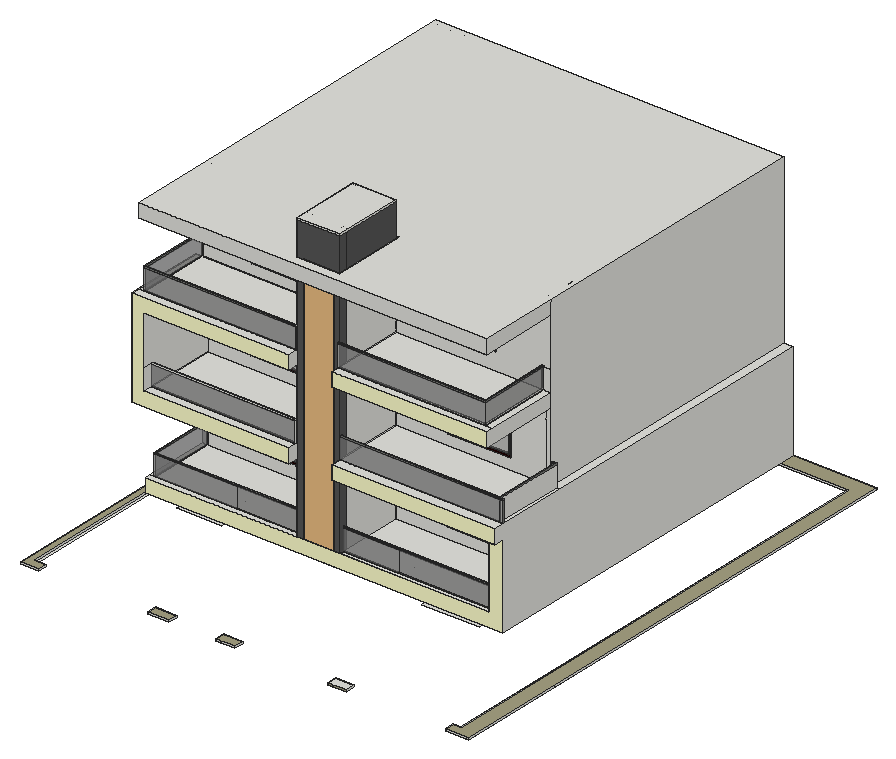
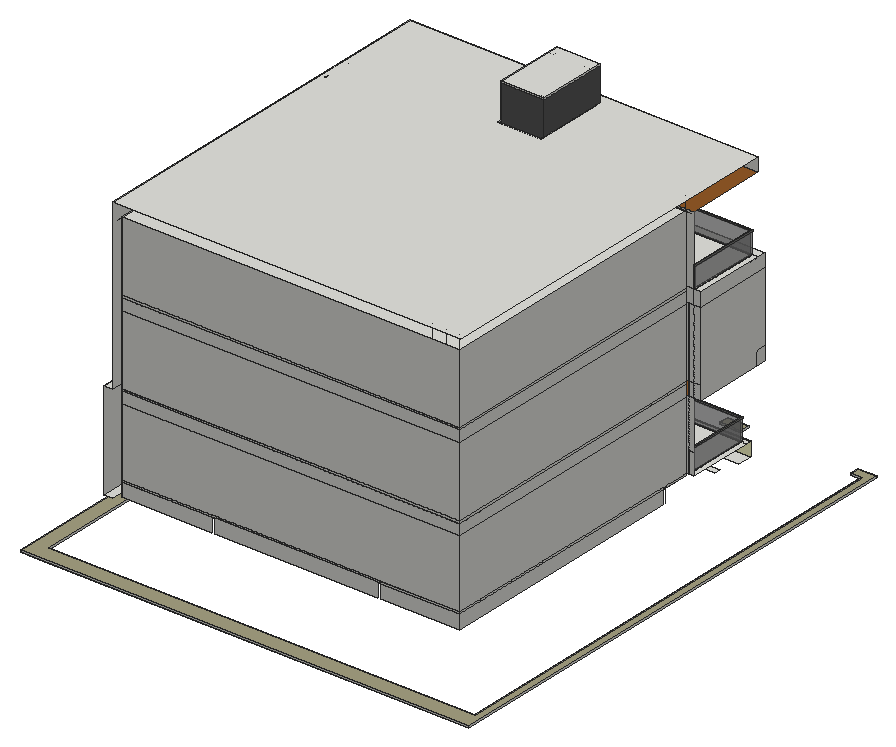
# SketchUp Ruby script. Lengths in inches.
U = 1.inch
M = Sketchup.active_model
def pt(a) = Geom::Point3d.new(a.map { |v| v * U })
def face(e, loops, mat)
  f = e.add_face(loops[0].map { |a| pt(a) })
  loops[1..].each { |l| e.add_face(l.map { |a| pt(a) }).erase! }
  f.material = f.back_material = mat if mat
  f
end
# faces: each face lists its corners as indices into pts; further lists are holes
def faces(e, pts, list, mat = nil) = list.each { |f| face(e, (f[0].is_a?(Array) ? f : [f]).map { |l| l.map { |i| pts[i] } }, mat) }
# xy, xz, yz: faces in a plane at the given z, y or x. An outline is a flat list of corners, or four numbers for a rectangle; further outlines are holes
def ring(l) = l.size == 4 ? [[l[0], l[1]], [l[2], l[1]], [l[2], l[3]], [l[0], l[3]]] : l.each_slice(2).to_a
def flat(e, list, mat, &to3) = list.each { |f| face(e, (f[0].is_a?(Array) ? f : [f]).map { |l| ring(l).map { |u, v| to3.(u, v) } }, mat) }
def xy(e, z, list, mat = nil) = flat(e, list, mat) { |x, y| [x, y, z] }
def xz(e, y, list, mat = nil) = flat(e, list, mat) { |x, z| [x, y, z] }
def yz(e, x, list, mat = nil) = flat(e, list, mat) { |y, z| [x, y, z] }
def lines(e, pts, list) = list.each { |a, b| e.add_line(pt(pts[a]), pt(pts[b])) }
# prism: a flat outline (further loops are holes) pulled along v
def prism(e, loops, v, mat = nil)
  f = face(e, loops, mat); d = Geom::Vector3d.new(v.map { |x| x * U })
  f.pushpull(f.normal.samedirection?(d) ? d.length : -d.length)
end
def box(e, o, s, mat = nil) = prism(e, [[o, [o[0] + s[0], o[1], o[2]], [o[0] + s[0], o[1] + s[1], o[2]], [o[0], o[1] + s[1], o[2]]]], [0, 0, s[2]], mat)
def at(x, y, z, deg = 0) = Geom::Transformation.translation(pt([x, y, z])) * Geom::Transformation.rotation(ORIGIN, Z_AXIS, deg.degrees)
def axes(o, x, y, z) = Geom::Transformation.new([*x, 0, *y, 0, *z, 0, *pt(o).to_a, 1])
def part(name) = M.definitions.add(name)
# library, detail: a bought-in or finely detailed component or shape, given as its bounding box
def library(name, o, s) = part(name).tap { |d| box(d.entities, o, s) }
def detail(e, o, s) = box(e.add_group.entities, o, s)
def put(e, d, t, mat = nil) = e.add_instance(d, t).tap { |i| i.material = mat if mat }
def group(e, t, mat = nil) = e.add_group.tap { |g| g.transformation = t; g.material = mat if mat }.entities
root = M.entities
M.materials.add("[Color A08]").color = [30, 0, 0]
M.materials.add("[Color E01]").color = [255, 255, 204]
M.materials.add("[Color M06]").color = [86, 86, 86]
M.materials.add("[Metal Seamed]").color = [118, 119, 115]
M.materials.add("[Stone Coursed Rough]").color = [165, 160, 130]
M.materials.add("[Translucent Glass Gray]").color = [128, 128, 128]
M.materials["[Translucent Glass Gray]"].alpha = 0.5
M.materials.add("[Wood Floor Parquet]").color = [145, 89, 39]
c1 = library("Group\#4",[0,0,0],[132.0625,6,363.3125])
c2 = part("Group\#3")
xy(c2.entities,0,[[0,0,60.375,4]])
xy(c2.entities,4.67,[[4.67,0,28.45,4],[32.75,0,55.71,4]],"[Color A08]")
xy(c2.entities,93.02,[[4.67,0,28.45,4],[32.75,0,55.71,4]])
xy(c2.entities,97.6875,[[0,0,60.375,4]],"[Color A08]")
xz(c2.entities,0,[[[0,0,60.375,97.6875],[4.67,4.67,28.45,93.02],[32.75,4.67,55.71,93.02]]],"[Color A08]")
xz(c2.entities,0,[[4.67,4.67,28.45,93.02],[32.75,4.67,55.71,93.02]],"[Translucent Glass Gray]")
xz(c2.entities,4,[[[0,0,60.375,97.6875],[4.67,4.67,28.45,93.02],[32.75,4.67,55.71,93.02]]],"[Color A08]")
yz(c2.entities,0,[[0,0,4,97.6875]],"[Color A08]")
yz(c2.entities,4.67,[[0,4.67,4,93.02]],"[Color A08]")
yz(c2.entities,28.45,[[0,4.67,4,93.02]],"[Color A08]")
yz(c2.entities,32.75,[[0,4.67,4,93.02]],"[Color A08]")
yz(c2.entities,55.71,[[0,4.67,4,93.02]],"[Color A08]")
yz(c2.entities,60.375,[[0,0,4,97.6875]],"[Color A08]")
c3 = part("Group\#2")
xy(c3.entities,0,[[0,0,95.3125,6]])
xy(c3.entities,4.01,[[4.01,0,28.72,6],[32.91,0,56.47,6],[60.66,0,91.31,6]],"[Color A08]")
xy(c3.entities,82.62,[[4.01,0,28.72,6],[32.91,0,56.47,6],[60.66,0,91.31,6]])
xy(c3.entities,86.625,[[0,0,95.3125,6]],"[Color A08]")
xz(c3.entities,0,[[[0,0,95.3125,86.625],[60.66,4.01,91.31,82.62],[4.01,4.01,28.72,82.62],[32.91,4.01,56.47,82.62]]],"[Color A08]")
xz(c3.entities,0,[[4.01,4.01,28.72,82.62],[32.91,4.01,56.47,82.62],[60.66,4.01,91.31,82.62]],"[Translucent Glass Gray]")
xz(c3.entities,6,[[[0,0,95.3125,86.625],[60.66,4.01,91.31,82.62],[4.01,4.01,28.72,82.62],[32.91,4.01,56.47,82.62]]],"[Color A08]")
yz(c3.entities,0,[[0,0,6,86.625]],"[Color A08]")
yz(c3.entities,4.01,[[0,4.01,6,82.62]],"[Color A08]")
yz(c3.entities,28.72,[[0,4.01,6,82.62]],"[Color A08]")
yz(c3.entities,32.91,[[0,4.01,6,82.62]],"[Color A08]")
yz(c3.entities,56.47,[[0,4.01,6,82.62]],"[Color A08]")
yz(c3.entities,60.66,[[0,4.01,6,82.62]],"[Color A08]")
yz(c3.entities,91.31,[[0,4.01,6,82.62]],"[Color A08]")
yz(c3.entities,95.3125,[[0,0,6,86.625]],"[Color A08]")
xy(root,126,[[0,0,0,878.5,746.625,878.5,746.625,849.54,11.8,849.54,11.8,16.17,31.52,16.17,31.52,0],[219.71,0,256.64,16.17],[336.85,0,370.02,16.17],[529.83,0,562.05,16.17],[732.77,0,732.77,16.17,746.625,16.17,746.625,183.0625,772,183.0625,772,0],
  [11.8,16.17,16.36,849.54],[746.625,183.0625,772,849.54],[746.625,849.54,772,878.5]])
xy(root,129,[[529.83,0,562.05,16.17]])
xy(root,129,[[0,0,31.52,0,31.52,16.17,11.8,16.17,11.8,849.54,746.625,849.54,746.625,16.17,732.77,16.17,732.77,0,772,0,772,878.5,0,878.5],[219.71,0,256.64,16.17],[336.85,0,370.02,16.17]],"[Stone Coursed Rough]")
xy(root,160.875,[[269.59,330.0625,317.59,336.0625],[446.24,330.0625,494.24,336.0625]])
xy(root,174.47,[[362.91,203.5,408.97,209.5625]])
xy(root,174.78,[[545.68,183.0625,644.56,192.0625]])
xy(root,175.07,[[124.03,183.0625,201.03,192.0625]])
xy(root,196.875,[[89.625,159.1875,239.625,183.0625],[348.1875,159.1875,360.82,183.0625],[360.82,159.1875,360.82,192.0625,348.1875,192.0625,348.1875,203.5,422.35,203.5,422.35,192.0625,412.84,192.0625,412.84,159.1875],[412.84,159.1875,422.35,183.0625],[519.875,159.1875,704.125,183.0625],
  [689.625,183.0625,704.125,783.0625]])
xy(root,196.875,[[239.625,159.1875,348.1875,330.0625],[422.35,159.1875,519.875,330.0625]],"[Wood Floor Parquet]")
xy(root,220.875,[[89.625,159.1875,348.1875,166.875],[348.1875,159.1875,360.82,175.5625],[360.82,159.1875,412.84,168.1875],[412.84,159.1875,422.35,159.1875,412.84,161.125],[422.35,159.1875,680.625,159.1875,680.625,165.3,422.36,165.72],
  [680.625,165.3,422.36,165.72,422.37,168.1875,680.625,168.1875],[89.625,166.875,97,281.125],[97,166.875,97,281.125,98.625,281.125,98.625,168.1875,348.1875,168.1875,348.1875,166.875],[98.625,168.1875,348.1875,281.125],[360.82,168.1875,412.84,178.89],
  [422.37,168.1875,680.625,168.1875,680.625,281.125,422.38,281.125,422.38,175.5625],[348.1875,175.5625,348.1875,281.125,418.5,281.125,418.5,277.79,351.52,277.79,351.52,178.89,360.82,178.89,360.82,175.5625],[412.84,175.5625,412.84,178.89,419.05,178.89,419.05,277.79,418.5,277.79,418.5,281.125,422.38,281.125,422.38,175.5625],[351.52,178.89,419.05,277.79],[348.1875,281.125,351.23,287.125],
  [351.23,281.125,418.5,287.125],[418.5,281.125,422.38,287.125],[98.625,287.125,98.625,774.0625,680.625,774.0625,680.625,287.125,418.5,287.125,418.5,336.0625,351.23,336.0625,351.23,287.125],[351.23,287.125,418.5,336.0625]])
xy(root,223.875,[[98.625,287.125,680.625,774.0625]])
xy(root,233.21,[[370.73,277.79,406.73,284.92]])
xy(root,238.59,[[511.46,281.125,620.96,287.125]])
xy(root,242.34,[[172.09,281.125,281.59,287.125]])
xy(root,256.875,[[680.625,165.3,422.36,165.72,422.37,168.1875,680.625,168.1875],[97,166.875,97,281.125,98.625,281.125,98.625,168.1875,348.1875,168.1875,348.1875,166.875]])
xy(root,258.875,[[680.625,165.3,680.625,168.1875,422.37,168.1875,422.36,165.72],[97,166.875,348.1875,166.875,348.1875,168.1875,98.625,168.1875,98.625,281.125,97,281.125]],"[Metal Seamed]")
xy(root,317.21,[[370.73,277.79,406.73,284.92]])
xy(root,320.22,[[511.46,281.125,620.96,287.125]])
xy(root,323.97,[[172.09,281.125,281.59,287.125]])
xy(root,340.875,[[78.1875,142.25,78.1875,159.1875,98.625,159.1875,98.625,281.125,348.1875,281.125,348.1875,142.25],[422.38,142.25,422.38,281.125,680.625,281.125,680.625,159.1875,704.125,159.1875,704.125,142.25],[78.1875,159.1875,89.625,281.125],[89.625,159.1875,98.625,281.125]],"[Wood Floor Parquet]")
xy(root,360.875,[[98.625,287.125,680.625,774.0625]])
xy(root,364.875,[[98.625,142.25,348.1875,156.75],[422.38,142.25,704.125,159.3125],[98.625,156.75,348.1875,159.1875],[98.625,159.1875,348.1875,281.125],[422.38,159.3125,704.125,161],
  [422.38,161,696.47,281.125],[696.47,161,696.47,281.125,689.625,281.125,689.625,282.2,698.1875,282.2,698.1875,161],[698.1875,161,704.125,283.32],[689.625,282.2,698.1875,282.2,698.1875,283.32,704.125,283.32,704.125,783.0625,689.625,783.0625],[98.625,287.125,680.625,774.0625]])
xy(root,383.59,[[172.09,281.125,281.59,287.125],[511.46,281.125,620.96,287.125]])
xy(root,390.46,[[370.73,277.79,406.73,286.23]])
xy(root,400.875,[[98.625,156.75,348.1875,159.1875],[422.38,159.3125,704.125,161],[696.47,161,696.47,281.125,689.625,281.125,689.625,282.2,698.1875,282.2,698.1875,161]])
xy(root,402.875,[[98.625,156.75,348.1875,159.1875]])
xy(root,402.875,[[422.38,159.3125,704.125,161],[696.47,161,698.1875,161,698.1875,282.2,689.625,282.2,689.625,281.125,696.47,281.125]],"[Metal Seamed]")
xy(root,465.22,[[172.09,281.125,281.59,287.125],[511.46,281.125,620.96,287.125]])
xy(root,474.46,[[370.73,277.79,406.73,286.23]])
xy(root,484.875,[[98.625,142.25,348.1875,281.125],[422.38,142.25,689.625,281.125]],"[Wood Floor Parquet]")
xy(root,504.875,[[98.625,287.125,680.625,774.0625]])
xy(root,508.875,[[78.1875,142.25,78.1875,156.3125,87.1875,156.3125,87.1875,157.5,348.1875,157.5,348.1875,142.25],[422.38,142.25,689.625,155.5625],[422.38,155.5625,422.38,158.91,674.27,158.91,674.27,281.125,677.375,281.125,677.375,155.5625],[677.375,155.5625,689.625,281.125],[78.1875,156.3125,87.1875,281.125],
  [87.1875,157.5,87.1875,281.125,89.625,281.125,89.625,159.1875,348.1875,159.1875,348.1875,157.5],[422.38,158.91,674.27,281.125],[89.625,159.1875,348.1875,281.125],[98.625,287.125,680.625,774.0625]])
xy(root,526.4,[[173.42,281.125,250.74,287.125]])
xy(root,534.65,[[370.73,277.79,406.73,281.125]])
xy(root,538.85,[[540.17,281.125,594.55,287.125]])
xy(root,544.875,[[422.38,155.5625,422.38,158.91,674.27,158.91,674.27,281.125,677.375,281.125,677.375,155.5625],[87.1875,157.5,87.1875,281.125,89.625,281.125,89.625,159.1875,348.1875,159.1875,348.1875,157.5]])
xy(root,546.875,[[422.38,155.5625,677.375,155.5625,677.375,281.125,674.27,281.125,674.27,158.91,422.38,158.91],[87.1875,157.5,348.1875,157.5,348.1875,159.1875,89.625,159.1875,89.625,281.125,87.1875,281.125]],"[Metal Seamed]")
xy(root,603.71,[[173.42,281.125,250.74,287.125]])
xy(root,608.22,[[540.17,281.125,594.55,287.125]])
xy(root,618.65,[[370.73,277.79,406.73,281.125]])
xy(root,628.875,[[348.1875,142.25,422.38,159.1875],[98.625,287.125,680.625,774.0625]])
xy(root,628.875,[[89.625,142.25,348.1875,281.125],[422.38,142.25,689.625,281.125]],"[Wood Floor Parquet]")
xy(root,652.875,[[[89.625,142.25,689.625,783.0625],[348.1875,159.1875,422.38,287.125]],[360.82,159.1875,412.84,178.89]])
xy(root,710.125,[[348.1875,159.1875,360.82,175.5625],[360.82,159.1875,412.84,175.5625],[412.84,159.1875,412.84,175.5625,422.38,175.5625,422.35,159.1875],[422.35,159.1875,422.38,175.5625,422.38,159.1875],[[348.1875,175.5625,422.38,281.125],[351.52,178.89,419.05,277.79]]])
xy(root,713.125,[[348.1875,159.1875,422.38,281.125]])
xz(root,0,[[0,126,31.52,129],[219.71,126,256.64,129],[336.85,126,370.02,129],[732.77,126,772,129]])
xz(root,0,[[529.83,126,562.05,129]],"[Stone Coursed Rough]")
xz(root,16.17,[[11.8,126,31.52,129],[219.71,126,256.64,129],[336.85,126,370.02,129],[529.83,126,562.05,129],[732.77,126,746.625,129]])
xz(root,142.25,[[89.625,628.875,689.625,652.875]])
xz(root,142.25,[[78.1875,340.875,348.1875,340.875,348.1875,364.875,98.625,364.875,98.625,484.875,348.1875,484.875,348.1875,508.875,78.1875,508.875],[422.38,340.875,704.125,364.875],[422.38,484.875,689.625,508.875]],"[Color E01]")
xz(root,155.5625,[[422.38,544.875,677.375,546.875]],"[Metal Seamed]")
xz(root,155.5625,[[422.38,508.875,677.375,544.875]],"[Translucent Glass Gray]")
xz(root,156.75,[[98.625,400.875,348.1875,402.875]])
xz(root,156.75,[[98.625,364.875,348.1875,400.875]],"[Translucent Glass Gray]")
xz(root,157.5,[[87.1875,544.875,348.1875,546.875]],"[Metal Seamed]")
xz(root,157.5,[[87.1875,508.875,348.1875,544.875]],"[Translucent Glass Gray]")
xz(root,158.91,[[422.38,544.875,674.27,546.875]],"[Metal Seamed]")
xz(root,158.91,[[422.38,508.875,674.27,544.875]],"[Translucent Glass Gray]")
xz(root,159.1875,[[78.1875,340.875,98.625,364.875],[98.625,400.875,348.1875,402.875],[360.82,628.875,412.84,652.875],[412.84,628.875,422.35,652.875],[422.35,628.875,422.38,652.875],
  [348.1875,710.125,422.38,713.125]])
xz(root,159.1875,[[89.625,196.875,704.125,196.875,704.125,340.875,680.625,340.875,680.625,220.875,89.625,220.875]],"[Color E01]")
xz(root,159.1875,[[348.1875,220.875,360.82,628.875],[412.84,220.875,422.35,628.875],[348.1875,652.875,422.35,710.125]],"[Color M06]")
xz(root,159.1875,[[89.625,544.875,348.1875,546.875]],"[Metal Seamed]")
xz(root,159.1875,[[98.625,364.875,348.1875,400.875],[89.625,508.875,348.1875,544.875]],"[Translucent Glass Gray]")
xz(root,159.3125,[[422.38,400.875,704.125,402.875]],"[Metal Seamed]")
xz(root,159.3125,[[422.38,364.875,704.125,400.875]],"[Translucent Glass Gray]")
xz(root,161,[[696.47,364.875,698.1875,400.875],[698.1875,364.875,704.125,400.875]])
xz(root,161,[[422.38,400.875,696.47,402.875],[696.47,400.875,698.1875,402.875],[698.1875,400.875,704.125,402.875]],"[Metal Seamed]")
xz(root,161,[[422.38,364.875,696.47,400.875]],"[Translucent Glass Gray]")
xz(root,166.875,[[97,256.875,348.1875,258.875]],"[Metal Seamed]")
xz(root,166.875,[[97,220.875,348.1875,256.875]],"[Translucent Glass Gray]")
xz(root,168.1875,[[239.625,256.875,348.1875,258.875],[519.875,256.875,680.625,258.875]])
xz(root,168.1875,[[98.625,256.875,239.625,258.875],[422.37,256.875,519.875,258.875]],"[Metal Seamed]")
xz(root,168.1875,[[98.625,220.875,239.625,256.875],[239.625,220.875,348.1875,256.875],[422.37,220.875,519.875,256.875],[519.875,220.875,680.625,256.875]],"[Translucent Glass Gray]")
xz(root,175.5625,[[412.84,220.875,422.38,710.125]])
xz(root,178.89,[[351.52,220.875,360.82,710.125],[412.84,220.875,419.05,710.125],[360.82,652.875,412.84,710.125]])
xz(root,277.79,[[[351.52,220.875,419.05,710.125],[370.73,534.65,406.73,618.65],[370.73,390.46,406.73,474.46],[370.73,233.21,406.73,317.21]]])
xz(root,281.125,[[89.625,220.875,97,256.875],[97,220.875,98.625,256.875],[[98.625,220.875,348.1875,340.875],[172.09,242.34,281.59,323.97]],[[422.38,220.875,680.625,340.875],[511.46,238.59,620.96,320.22]],[89.625,256.875,97,256.875,97,258.875,98.625,258.875,98.625,340.875,89.625,340.875],
  [97,256.875,98.625,258.875],[78.1875,340.875,89.625,364.875],[89.625,340.875,98.625,364.875],[78.1875,364.875,89.625,484.875],[89.625,364.875,98.625,484.875],
  [[98.625,364.875,348.1875,484.875],[172.09,383.59,281.59,465.22]],[[422.38,364.875,680.625,484.875],[511.46,383.59,620.96,465.22]],[680.625,364.875,689.625,484.875],[689.625,364.875,696.47,400.875],[689.625,400.875,696.47,402.875],
  [78.1875,484.875,89.625,508.875],[89.625,484.875,348.1875,508.875],[87.1875,508.875,89.625,544.875],[[89.625,508.875,348.1875,628.875],[173.42,526.4,250.74,603.71]],[[422.38,508.875,674.27,508.875,674.27,546.875,677.375,546.875,677.375,544.875,689.625,544.875,689.625,628.875,422.38,628.875],[540.17,538.85,594.55,608.22]],
  [674.27,508.875,677.375,544.875],[677.375,508.875,689.625,544.875],[87.1875,544.875,89.625,546.875],[674.27,544.875,677.375,546.875],[348.1875,710.125,422.38,713.125]])
xz(root,281.125,[[[348.1875,220.875,422.38,710.125],[370.73,534.65,406.73,618.65]]],"[Color M06]")
xz(root,282.2,[[689.625,364.875,698.1875,400.875],[689.625,400.875,698.1875,402.875]],"[Metal Seamed]")
xz(root,284.92,[[370.73,233.21,406.73,317.21]])
xz(root,286.23,[[370.73,390.46,406.73,474.46]])
xz(root,287.125,[[98.625,220.875,348.1875,223.875],[348.1875,220.875,422.38,223.875],[422.38,220.875,680.625,223.875],[[98.625,223.875,348.1875,340.875],[172.09,242.34,281.59,323.97]],[348.1875,223.875,422.38,360.875],
  [[422.38,223.875,680.625,340.875],[511.46,238.59,620.96,320.22]],[98.625,340.875,348.1875,360.875],[422.38,340.875,680.625,360.875],[98.625,360.875,348.1875,364.875],[348.1875,360.875,422.38,364.875],
  [422.38,360.875,643.3,364.875],[643.3,360.875,670.11,364.875],[670.11,360.875,680.625,364.875],[[98.625,364.875,348.1875,484.875],[172.09,383.59,281.59,465.22]],[348.1875,364.875,422.38,504.875],
  [[422.38,364.875,680.625,484.875],[511.46,383.59,620.96,465.22]],[98.625,484.875,348.1875,504.875],[422.38,484.875,680.625,504.875],[98.625,504.875,348.1875,508.875],[348.1875,504.875,422.38,508.875],
  [422.38,504.875,680.625,508.875],[[98.625,508.875,348.1875,628.875],[173.42,526.4,250.74,603.71]],[348.1875,508.875,422.38,628.875],[[422.38,508.875,680.625,628.875],[540.17,538.85,594.55,608.22]],[348.1875,628.875,422.38,652.875]])
xz(root,774.0625,[[98.625,196.875,233.625,220.875],[239.625,196.875,519.875,220.875],[525.875,196.875,680.625,220.875],[98.625,220.875,233.625,223.875],[233.625,220.875,239.625,223.875],
  [239.625,220.875,519.875,223.875],[519.875,220.875,525.875,223.875],[525.875,220.875,680.625,223.875],[98.625,223.875,680.625,340.875],[98.625,340.875,680.625,360.875],
  [98.625,360.875,680.625,364.875],[98.625,364.875,680.625,484.875],[98.625,484.875,680.625,504.875],[98.625,504.875,680.625,508.875],[98.625,508.875,680.625,628.875]])
xz(root,849.54,[[11.8,126,746.625,129]])
xz(root,878.5,[[0,126,772,129]])
yz(root,0,[[0,126,878.5,129]])
yz(root,11.8,[[16.17,126,849.54,129]])
yz(root,31.52,[[0,126,16.17,129]])
yz(root,78.1875,[[142.25,340.875,159.1875,364.875],[159.1875,340.875,159.1875,364.875,142.25,364.875,142.25,484.875,281.125,484.875,281.125,340.875],[142.25,484.875,281.125,508.875]])
yz(root,87.1875,[[157.5,544.875,281.125,546.875]],"[Metal Seamed]")
yz(root,87.1875,[[157.5,508.875,281.125,544.875]],"[Translucent Glass Gray]")
yz(root,89.625,[[159.1875,544.875,281.125,546.875]],"[Metal Seamed]")
yz(root,89.625,[[159.1875,508.875,281.125,544.875]],"[Translucent Glass Gray]")
yz(root,97,[[166.875,256.875,281.125,258.875]],"[Metal Seamed]")
yz(root,97,[[166.875,220.875,281.125,256.875]],"[Translucent Glass Gray]")
yz(root,98.625,[[336.0625,196.875,774.0625,220.875],[287.125,220.875,330.0625,223.875],[330.0625,220.875,336.0625,223.875],[336.0625,220.875,774.0625,223.875],[287.125,223.875,774.0625,340.875],
  [159.1875,340.875,281.125,364.875],[287.125,340.875,774.0625,360.875],[287.125,360.875,327.41,364.875],[327.41,360.875,362.35,364.875],[362.35,360.875,774.0625,364.875],
  [142.25,364.875,156.75,400.875],[159.1875,364.875,281.125,364.875,281.125,484.875,142.25,484.875,142.25,400.875,156.75,400.875,156.75,402.875,159.1875,402.875],[156.75,364.875,159.1875,400.875],[287.125,364.875,774.0625,484.875],[156.75,400.875,159.1875,402.875],
  [287.125,484.875,774.0625,504.875],[287.125,504.875,774.0625,508.875],[287.125,508.875,774.0625,628.875]])
yz(root,98.625,[[168.1875,256.875,281.125,258.875]],"[Metal Seamed]")
yz(root,98.625,[[168.1875,220.875,281.125,256.875]],"[Translucent Glass Gray]")
yz(root,172.09,[[281.125,242.34,287.125,323.97],[281.125,383.59,287.125,465.22]])
yz(root,173.42,[[281.125,526.4,287.125,603.71]])
yz(root,219.71,[[0,126,16.17,129]])
yz(root,250.74,[[281.125,526.4,287.125,603.71]])
yz(root,256.64,[[0,126,16.17,129]])
yz(root,281.59,[[281.125,242.34,287.125,323.97],[281.125,383.59,287.125,465.22]])
yz(root,336.85,[[0,126,16.17,129]])
yz(root,348.1875,[[159.1875,220.875,166.875,256.875],[166.875,220.875,168.1875,256.875],[168.1875,220.875,175.5625,340.875],[175.5625,220.875,281.125,340.875],[281.125,220.875,287.125,340.875],
  [159.1875,256.875,159.1875,340.875,168.1875,340.875,168.1875,258.875,166.875,258.875,166.875,256.875],[166.875,256.875,168.1875,258.875],[142.25,340.875,159.1875,364.875],[159.1875,340.875,168.1875,364.875],[168.1875,340.875,175.5625,364.875],
  [175.5625,340.875,281.125,364.875],[281.125,340.875,287.125,364.875],[156.75,364.875,159.1875,400.875],[159.1875,364.875,168.1875,484.875],[168.1875,364.875,175.5625,484.875],
  [175.5625,364.875,281.125,484.875],[281.125,364.875,287.125,484.875],[156.75,400.875,159.1875,402.875],[142.25,484.875,159.1875,508.875],[159.1875,484.875,168.1875,508.875],
  [168.1875,484.875,175.5625,508.875],[175.5625,484.875,281.125,508.875],[281.125,484.875,287.125,508.875],[157.5,508.875,159.1875,544.875],[168.1875,508.875,175.5625,628.875],
  [175.5625,508.875,281.125,628.875],[281.125,508.875,287.125,628.875],[157.5,544.875,159.1875,546.875],[168.1875,628.875,175.5625,652.875],[175.5625,628.875,281.125,652.875],
  [281.125,628.875,287.125,652.875],[159.1875,710.125,281.125,713.125]])
yz(root,348.1875,[[159.1875,508.875,168.1875,628.875],[159.1875,652.875,281.125,710.125]],"[Color M06]")
yz(root,351.23,[[209.5625,196.875,336.0625,220.875]])
yz(root,351.52,[[178.89,220.875,277.79,710.125]])
yz(root,360.82,[[159.1875,220.875,168.1875,652.875],[168.1875,220.875,175.4375,652.875],[175.4375,220.875,175.5625,652.875],[175.5625,220.875,178.89,652.875],[168.1875,652.875,175.4375,710.125],
  [175.4375,652.875,175.5625,710.125]])
yz(root,370.02,[[0,126,16.17,129]])
yz(root,370.73,[[277.79,233.21,284.92,317.21],[277.79,390.46,286.23,474.46],[277.79,534.65,281.125,618.65]])
yz(root,406.73,[[277.79,233.21,284.92,317.21],[277.79,390.46,286.23,474.46],[277.79,534.65,281.125,618.65]])
yz(root,412.84,[[159.1875,220.875,161.125,652.875],[161.125,220.875,168.1875,652.875],[168.1875,220.875,175.5625,652.875],[175.5625,220.875,178.89,652.875]])
yz(root,418.5,[[209.5625,196.875,336.0625,220.875]])
yz(root,419.05,[[178.89,220.875,277.79,710.125]])
yz(root,422.38,[[175.5625,220.875,281.125,340.875],[281.125,220.875,287.125,340.875],[142.25,340.875,175.5625,364.875],[175.5625,340.875,281.125,364.875],[281.125,340.875,287.125,364.875],
  [159.3125,364.875,161,400.875],[175.5625,364.875,281.125,484.875],[281.125,364.875,287.125,484.875],[159.3125,400.875,161,402.875],[142.25,484.875,175.5625,508.875],
  [175.5625,484.875,281.125,508.875],[281.125,484.875,287.125,508.875],[155.5625,508.875,158.91,544.875],[175.5625,508.875,281.125,625.1875],[281.125,508.875,287.125,628.875],
  [155.5625,544.875,158.91,546.875],[175.5625,625.1875,281.125,628.875],[159.1875,628.875,175.5625,652.875],[175.5625,628.875,281.125,652.875],[281.125,628.875,287.125,652.875],
  [159.1875,710.125,281.125,713.125]])
yz(root,422.38,[[175.5625,652.875,281.125,710.125]],"[Color M06]")
yz(root,511.46,[[281.125,238.59,287.125,320.22],[281.125,383.59,287.125,465.22]])
yz(root,529.83,[[0,126,16.17,129]])
yz(root,540.17,[[281.125,538.85,287.125,608.22]])
yz(root,562.05,[[0,126,16.17,129]])
yz(root,594.55,[[281.125,538.85,287.125,608.22]])
yz(root,620.96,[[281.125,238.59,287.125,320.22],[281.125,383.59,287.125,465.22]])
yz(root,674.27,[[158.91,544.875,281.125,546.875]],"[Metal Seamed]")
yz(root,674.27,[[158.91,508.875,281.125,544.875]],"[Translucent Glass Gray]")
yz(root,677.375,[[155.5625,544.875,281.125,546.875]],"[Metal Seamed]")
yz(root,677.375,[[155.5625,508.875,281.125,544.875]],"[Translucent Glass Gray]")
yz(root,680.625,[[336.0625,196.875,774.0625,220.875],[159.1875,220.875,159.1875,340.875,192.0625,340.875,192.0625,220.875,168.1875,220.875,168.1875,258.875,165.3,258.875,165.3,220.875],[165.3,220.875,168.1875,256.875],[192.0625,220.875,281.125,340.875],[287.125,220.875,330.0625,223.875],
  [330.0625,220.875,336.0625,223.875],[336.0625,220.875,774.0625,223.875],[287.125,223.875,330.0625,340.875],[330.0625,223.875,336.0625,340.875],[336.0625,223.875,774.0625,340.875],
  [165.3,256.875,168.1875,258.875],[287.125,340.875,774.0625,360.875],[287.125,360.875,330.0625,364.875],[330.0625,360.875,336.0625,364.875],[336.0625,360.875,774.0625,364.875],
  [287.125,364.875,330.0625,484.875],[330.0625,364.875,336.0625,484.875],[336.0625,364.875,774.0625,504.875],[287.125,484.875,330.0625,504.875],[330.0625,484.875,336.0625,504.875],
  [287.125,504.875,330.0625,508.875],[330.0625,504.875,336.0625,508.875],[336.0625,504.875,774.0625,508.875],[287.125,508.875,330.0625,628.875],[330.0625,508.875,336.0625,628.875],
  [336.0625,508.875,774.0625,628.875],[330.0625,628.875,336.0625,652.875]])
yz(root,689.625,[[281.125,364.875,282.2,400.875],[282.2,364.875,783.0625,364.875,783.0625,652.875,281.125,652.875,281.125,402.875,282.2,402.875],[281.125,400.875,282.2,402.875],[142.25,484.875,281.125,508.875],[142.25,628.875,281.125,652.875]])
yz(root,696.47,[[161,364.875,281.125,400.875]])
yz(root,696.47,[[161,400.875,281.125,402.875]],"[Metal Seamed]")
yz(root,698.1875,[[161,364.875,282.2,400.875]])
yz(root,698.1875,[[161,400.875,282.2,402.875]],"[Metal Seamed]")
yz(root,704.125,[[159.1875,196.875,783.0625,196.875,783.0625,364.875,142.25,364.875,142.25,340.875,159.1875,340.875]])
yz(root,704.125,[[159.3125,364.875,161,400.875],[159.3125,400.875,161,402.875]],"[Metal Seamed]")
yz(root,732.77,[[0,126,16.17,129]])
yz(root,746.625,[[16.17,126,183.0625,129],[183.0625,126,849.54,129]])
yz(root,772,[[0,126,183.0625,129],[183.0625,126,878.5,129]])
p = [[422.36,165.72,258.875],[422.37,168.1875,258.875],[422.37,168.1875,256.875],[422.37,168.1875,220.875],[422.38,175.5625,220.875],[422.38,175.5625,340.875],
  [422.38,175.5625,364.875],[422.38,175.5625,484.875],[422.38,175.5625,508.875],[422.38,175.5625,625.1875],[422.38,175.5625,628.875],[422.38,175.5625,652.875],
  [422.38,175.5625,710.125],[422.35,159.1875,710.125],[422.35,159.1875,652.875],[422.35,159.1875,628.875],[422.35,159.1875,220.875],[422.36,165.72,220.875],
  [422.36,165.72,256.875],[680.625,165.3,220.875],[680.625,165.3,256.875],[680.625,165.3,258.875],[525.875,336.0625,196.875],[525.875,336.0625,220.875],
  [233.625,336.0625,196.875],[233.625,336.0625,220.875],[519.875,336.0625,196.875],[519.875,336.0625,220.875],[239.625,336.0625,196.875],[239.625,336.0625,220.875],
  [233.625,192.0625,196.875],[233.625,192.0625,220.875],[233.625,330.0625,196.875],[233.625,330.0625,220.875],[98.625,330.0625,196.875],[98.625,330.0625,220.875],
  [525.875,192.0625,196.875],[525.875,192.0625,220.875],[680.625,192.0625,196.875],[680.625,192.0625,220.875],[525.875,330.0625,196.875],[525.875,330.0625,220.875],
  [680.625,330.0625,196.875],[680.625,330.0625,220.875],[422.35,168.1875,220.875],[680.625,783.0625,628.875],[680.625,774.0625,628.875],[98.625,287.125,628.875],
  [89.625,287.125,628.875],[98.625,774.0625,628.875],[98.625,774.0625,652.875],[122,774.0625,628.875],[122,774.0625,652.875],[145.375,774.0625,628.875],
  [145.375,774.0625,652.875],[98.625,287.125,652.875],[680.625,287.125,628.875],[680.625,287.125,652.875],[412.84,175.5625,710.125],[412.84,175.5625,713.125],
  [351.52,277.79,710.125],[351.52,277.79,713.125],[355.71,277.79,710.125],[355.71,277.79,713.125],[351.52,178.89,710.125],[351.52,178.89,713.125],
  [360.82,178.89,710.125],[360.82,178.89,713.125],[412.84,178.89,710.125],[412.84,178.89,713.125],[419.05,178.89,710.125],[419.05,178.89,713.125],
  [419.05,277.79,710.125],[419.05,277.79,713.125]]
faces(root,p,[[0,1,2,3,4,5,6,7,8,9,10,11,12,13,14,15,16,17,18]],"[Color M06]")
faces(root,p,[[17,19,20,18]],"[Translucent Glass Gray]")
faces(root,p,[[17,3,2,18],[18,2,1,0]])
faces(root,p,[[18,20,21,0]],"[Metal Seamed]")
lines(root,p,[[22,23],[24,25],[26,27],[28,29],[30,31],[32,33],[34,35],[36,37],[38,39],[40,41],[42,43],[44,3],
  [45,46],[47,48],[49,50],[51,52],[53,54],[47,55],[56,57],[58,59],[60,61],[62,63],[64,65],[66,67],
  [68,69],[70,71],[72,73]])
put(root,c1,axes([360.82,159.1875,220.875],[0.39392,0,0],[0,0.8246,0],[0,0,1.123]))
put(root,c2,axes([370.55,277.86,233.21],[0.59917,0,0],[0,0.51652,0],[0,0,0.85987]))
put(root,c3,axes([511.33,281.125,238.59],[1.1502,0,0],[0,0.71,0],[0,0,0.94228]))
put(root,c3,axes([171.96,281.125,242.34],[1.1502,0,0],[0,0.71,0],[0,0,0.94228]))
put(root,c3,axes([511.33,281.125,383.59],[1.1502,0,0],[0,0.71,0],[0,0,0.94228]))
put(root,c3,axes([171.96,281.125,383.59],[1.1502,0,0],[0,0.71,0],[0,0,0.94228]))
put(root,c2,axes([370.55,277.86,390.46],[0.59917,0,0],[0,0.51652,0],[0,0,0.85987]))
put(root,c3,axes([173.42,281.125,526.4],[0.81115,0,0],[0,0.355,0],[0,0,0.8925]))
put(root,c2,axes([370.55,277.86,534.65],[0.59917,0,0],[0,0.51652,0],[0,0,0.85987]))
put(root,c3,axes([538.88,281.125,538.85],[0.58403,0,0],[0,0.213,0],[0,0,0.80087]))
